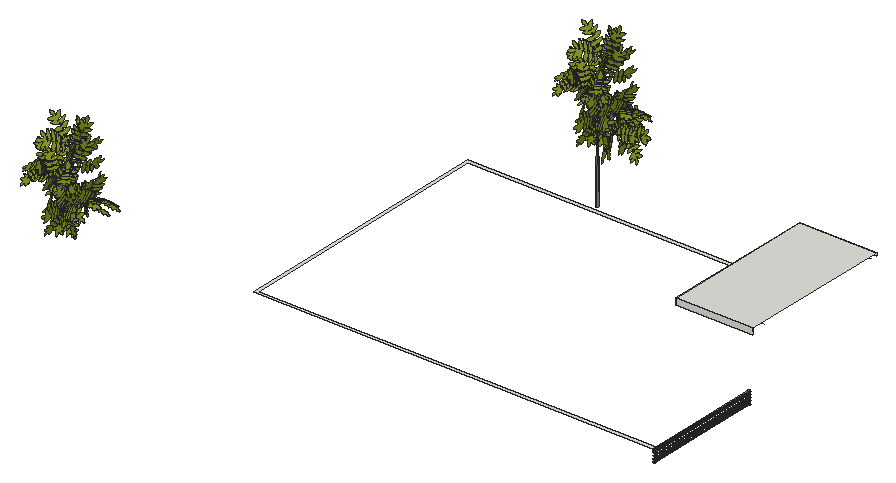
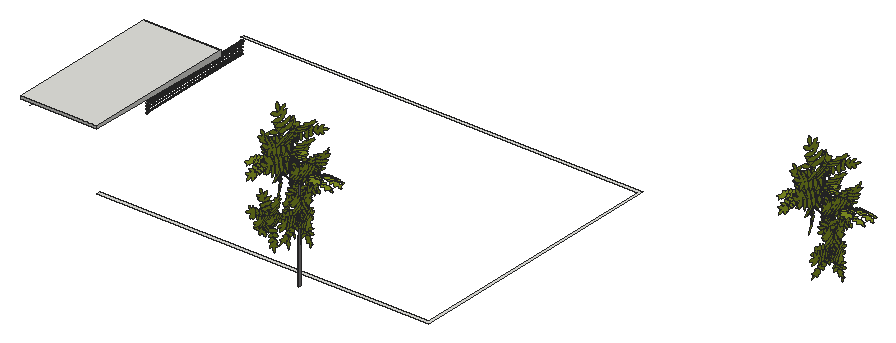
# SketchUp Ruby script. Lengths in inches.
U = 1.inch
M = Sketchup.active_model
def pt(a) = Geom::Point3d.new(a.map { |v| v * U })
def face(e, loops, mat)
  f = e.add_face(loops[0].map { |a| pt(a) })
  loops[1..].each { |l| e.add_face(l.map { |a| pt(a) }).erase! }
  f.material = f.back_material = mat if mat
  f
end
# faces: each face lists its corners as indices into pts; further lists are holes
def faces(e, pts, list, mat = nil) = list.each { |f| face(e, (f[0].is_a?(Array) ? f : [f]).map { |l| l.map { |i| pts[i] } }, mat) }
# xy, xz, yz: faces in a plane at the given z, y or x. An outline is a flat list of corners, or four numbers for a rectangle; further outlines are holes
def ring(l) = l.size == 4 ? [[l[0], l[1]], [l[2], l[1]], [l[2], l[3]], [l[0], l[3]]] : l.each_slice(2).to_a
def flat(e, list, mat, &to3) = list.each { |f| face(e, (f[0].is_a?(Array) ? f : [f]).map { |l| ring(l).map { |u, v| to3.(u, v) } }, mat) }
def xy(e, z, list, mat = nil) = flat(e, list, mat) { |x, y| [x, y, z] }
def xz(e, y, list, mat = nil) = flat(e, list, mat) { |x, z| [x, y, z] }
def yz(e, x, list, mat = nil) = flat(e, list, mat) { |y, z| [x, y, z] }
def lines(e, pts, list) = list.each { |a, b| e.add_line(pt(pts[a]), pt(pts[b])) }
# prism: a flat outline (further loops are holes) pulled along v
def prism(e, loops, v, mat = nil)
  f = face(e, loops, mat); d = Geom::Vector3d.new(v.map { |x| x * U })
  f.pushpull(f.normal.samedirection?(d) ? d.length : -d.length)
end
def box(e, o, s, mat = nil) = prism(e, [[o, [o[0] + s[0], o[1], o[2]], [o[0] + s[0], o[1] + s[1], o[2]], [o[0], o[1] + s[1], o[2]]]], [0, 0, s[2]], mat)
def at(x, y, z, deg = 0) = Geom::Transformation.translation(pt([x, y, z])) * Geom::Transformation.rotation(ORIGIN, Z_AXIS, deg.degrees)
def axes(o, x, y, z) = Geom::Transformation.new([*x, 0, *y, 0, *z, 0, *pt(o).to_a, 1])
def part(name) = M.definitions.add(name)
# library, detail: a bought-in or finely detailed component or shape, given as its bounding box
def library(name, o, s) = part(name).tap { |d| box(d.entities, o, s) }
def detail(e, o, s) = box(e.add_group.entities, o, s)
def put(e, d, t, mat = nil) = e.add_instance(d, t).tap { |i| i.material = mat if mat }
def group(e, t, mat = nil) = e.add_group.tap { |g| g.transformation = t; g.material = mat if mat }.entities
root = M.entities
M.materials.add("3D66_SU_1574822641685_001").color = [135, 150, 36]
M.materials.add("3D66_SU_1574822641883_002").color = [178, 165, 164]
M.materials.add("3D66_SU_1574822642012_003").color = [128, 125, 127]
M.materials.add("[Aluminum]").color = [150, 150, 150]
M.materials["[Aluminum]"].alpha = 0.5
c1 = part("rama-acacia")
p = [[-13.8,1.01,-1.08],[-13.61,0.91,-1.04],[-13.61,0.85,-1.06],[-14.07,0.85,-1.21],[-15.17,0.86,-1.58],[-15.95,0.92,-1.83],
  [-16.01,1,-1.83],[-16.01,1.17,-1.78],[-16.07,1.93,-1.6],[-16.4,2.73,-1.5],[-16.65,3.06,-1.5],[-17.13,4.01,-1.41],
  [-17.78,4.7,-1.44],[-18.28,5.07,-1.51],[-18.57,5.18,-1.58],[-18.91,5.47,-1.62],[-19.07,5.48,-1.67],[-19.35,5.61,-1.73],
  [-19.51,5.64,-1.78],[-19.38,5.57,-1.75],[-19.33,5.5,-1.75],[-19.31,5.23,-1.82],[-19.38,5.08,-1.89],[-19.41,4.84,-1.96],
  [-19.36,4.59,-2.01],[-19.43,4.55,-2.04],[-19.36,4.15,-2.125],[-19.21,3.7,-2.19],[-18.875,3.1,-2.24],[-18.61,2.78,-2.24],
  [-17.83,2.19,-2.13],[-17.4375,1.85,-2.09],[-17.04,1.49,-2.05],[-16.61,1.24,-1.97],[-16.17,1.0625,-1.87],[-16.06,0.95,-1.86],
  [-16.06,0.91,-1.87],[-16.32,0.9,-1.96],[-16.7,0.88,-2.1],[-17.05,0.91,-2.21],[-17.61,1.15,-2.33],[-18.06,1.29,-2.45],
  [-18.88,1.53,-2.67],[-20.25,1.46,-3.15],[-20.59,1.49,-3.26],[-20.79,1.37,-3.36],[-21.08,1.2,-3.5],[-21.28,1.22,-3.5625],
  [-21.48,0.94,-3.71],[-21.79,0.5,-3.93],[-22.02,0.17,-4.1],[-22.11,0.05,-4.16],[-22.21,-0.02,-4.21],[-22.375,-0.05,-4.28],
  [-22.375,-0.07,-4.28],[-22.18,-0.09,-4.22],[-22.11,-0.07,-4.19],[-21.78,-0.1,-4.09],[-21.6,-0.18,-4.05],[-21.52,-0.27,-4.04],
  [-21.33,-0.33,-4],[-20.94,-0.54,-3.92],[-20.6875,-0.63,-3.86],[-20.54,-0.68,-3.82],[-20.42,-0.67,-3.78],[-20.09,-0.46,-3.61],
  [-19.8,-0.24,-3.45],[-19.21,-0.02,-3.19],[-18.48,0.08,-2.92],[-17.72,0.38,-2.58],[-17.4,0.5,-2.4375],[-16.93,0.75,-2.21],
  [-16.78,0.8,-2.15],[-16.1,0.83,-1.91],[-16.0625,0.81,-1.9],[-16.08,0.77,-1.91],[-16.27,0.72,-1.99],[-16.88,0.39,-2.29],
  [-17.1875,0.15,-2.46],[-17.27,0.02,-2.52],[-17.94,-0.52,-2.89],[-17.94,-0.59,-2.91],[-18.08,-0.68,-2.99],[-18.13,-0.86,-3.05],
  [-18.56,-1.55,-3.38],[-18.71,-2.11,-3.58],[-18.79,-2.61,-3.74],[-18.86,-2.84,-3.83],[-18.87,-3.07,-3.89],[-18.84,-3.22,-3.92],
  [-18.8,-3.26,-3.92],[-18.76,-3.47,-3.96],[-18.76,-3.6,-4],[-18.67,-3.8,-4.02],[-18.61,-3.92,-4.04],[-18.58,-4.11,-4.07],
  [-18.53,-4.18,-4.08],[-18.58,-4.35,-4.14],[-18.65,-4.43,-4.18],[-18.72,-4.51,-4.23],[-18.8125,-4.51,-4.26],[-18.8125,-4.53,-4.26],
  [-18.72,-4.54,-4.24],[-18.66,-4.49,-4.21],[-18.58,-4.43,-4.16],[-18.35,-4.23,-4.03],[-18.32,-4.17,-4],[-18.22,-4.125,-3.95],
  [-18.1,-4,-3.88],[-17.79,-3.72,-3.7],[-17.68,-3.51,-3.61],[-17.32,-3.13,-3.38],[-17.24,-2.94,-3.31],[-16.78,-2.12,-2.93],
  [-16.48,-1.78,-2.73],[-16.3,-1.28,-2.54],[-16.05,-0.75,-2.3125],[-15.89,-0.2,-2.11],[-15.89,0.39,-1.95],[-15.96,0.79,-1.87],
  [-15.91,0.82,-1.84],[-15.27,0.8,-1.63],[-14.18,0.76,-1.27],[-13.78,0.73,-1.15],[-13.78,0.67,-1.16],[-14.23,0.54,-1.35],
  [-14.65,0.33,-1.55],[-14.97,0.02,-1.74],[-15.25,-0.36,-1.9375],[-15.57,-0.72,-2.14],[-15.96,-1.64,-2.52],[-16.2,-2.51,-2.84],
  [-16.2,-3.12,-3],[-16.14,-3.41,-3.06],[-16.1,-3.75,-3.14],[-16.1,-4.09,-3.23],[-16.2,-4.25,-3.3],[-16.2,-4.28,-3.3125],
  [-16.08,-4.19,-3.24],[-15.98,-4.08,-3.18],[-15.96,-3.94,-3.14],[-15.96,-3.8125,-3.1],[-15.9,-3.72,-3.06],[-15.68,-3.55,-2.9375],
  [-15.51,-3.49,-2.86],[-15.3,-3.33,-2.75],[-15.23,-3.17,-2.68],[-15.01,-3.03,-2.57],[-14.875,-2.83,-2.47],[-14.6,-2.59,-2.3125],
  [-14.4,-2.27,-2.16],[-14.12,-1.6,-1.89],[-13.91,-1.1,-1.68],[-13.67,-0.83,-1.53],[-13.53,-0.45,-1.38],[-13.53,0.67,-1.08],
  [-13.53,0.69,-1.07],[-13.38,0.86,-0.98],[-13.38,0.92,-0.96],[-13.32,1.03,-0.91],[-13.32,1.35,-0.82],[-13.28,1.49,-0.77],
  [-13.28,1.99,-0.64],[-13.44,2.67,-0.51],[-13.72,3.31,-0.43],[-13.93,3.71,-0.4],[-14.1,4.39,-0.27],[-14.5625,5.06,-0.25],
  [-14.89,5.62,-0.21],[-15.33,6.1,-0.23],[-15.65,6.8,-0.15],[-15.79,6.89,-0.18],[-15.61,6.52,-0.22],[-15.51,6.32,-0.24],
  [-15.45,6.28,-0.23],[-15.52,6,-0.32],[-15.63,5.6875,-0.45],[-15.77,4.97,-0.68],[-15.7,4.25,-0.85],[-15.46,3,-1.11],
  [-15,2.03,-1.21],[-14.3,1.29,-1.17],[-12.41,6.01,0.65],[-12.44,6.14,0.68],[-12.41,6.29,0.73],[-12.43,6.29,0.73],
  [-12.44,6.26,0.72],[-12.47,6.15,0.68],[-12.49,6.07,0.66],[-12.57,5.75,0.55],[-12.67,5.36,0.43],[-12.79,4.875,0.28],
  [-12.83,4.52,0.18],[-12.83,3.99,0.04],[-12.73,3.11,-0.18],[-12.58,2.52,-0.3125],[-12.3,1.97,-0.41],[-11.88,1.51,-0.46],
  [-11.37,1.0625,-0.48],[-10.75,0.75,-0.45],[-10.75,0.68,-0.47],[-12.55,0.7,-0.79],[-13.21,0.79,-0.89],[-13.2,0.67,-0.92],
  [-12.56,0.62,-0.82],[-11.15,0.56,-0.58],[-10.79,0.54,-0.52],[-10.72,0.52,-0.51],[-10.72,0.5,-0.52],[-10.87,0.47,-0.55],
  [-11.14,0.41,-0.62],[-11.39,0.27,-0.7],[-11.625,-0.01,-0.82],[-11.8,-0.43,-0.96],[-11.83,-0.57,-1],[-12.02,-1.08,-1.17],
  [-12.1,-1.39,-1.27],[-12.17,-1.95,-1.4375],[-12.17,-2.77,-1.65],[-12.09,-3.59,-1.86],[-11.86,-4.26,-2],[-11.8125,-4.4,-2.03],
  [-11.84,-4.49,-2.05],[-11.91,-4.6,-2.1],[-11.97,-4.65,-2.12],[-11.98,-4.67,-2.13],[-11.92,-4.65,-2.11],[-11.84,-4.59,-2.08],
  [-11.77,-4.52,-2.05],[-11.74,-4.47,-2.03],[-11.37,-4.3125,-1.92],[-10.95,-4.0625,-1.78],[-10.82,-3.89,-1.71],[-10.64,-3.57,-1.59],
  [-10.41,-3.05,-1.41],[-10.27,-2.73,-1.3],[-10.07,-1.88,-1.03],[-10.15,-0.71,-0.73],[-10.31,-0.1,-0.6],[-10.5,0.4,-0.5],
  [-10.5,0.48,-0.48],[-10.44,0.53,-0.45],[-10.39,0.64,-0.42],[-10.52,0.73,-0.42],[-10.44,0.93,-0.35],[-10.44,1.2,-0.28],
  [-10.32,1.47,-0.18],[-10.48,2.6875,0.12],[-10.43,2.96,0.2],[-10.75,3.87,0.38],[-11.26,4.93,0.57],[-11.8,5.54,0.64],
  [-12.37,5.93,0.64],[-7.78,0.19,-0.06],[-7.78,0.25,-0.04],[-7.75,0.39,0],[-7.89,0.4,-0.02],[-7.96,0.46,-0.02],
  [-7.96,0.49,-0.01],[-7.76,0.62,0.06],[-7.53,0.99,0.2],[-7.31,1.78,0.45],[-7.31,2.74,0.71],[-7.63,3.6875,0.9],
  [-8.02,4.57,1.07],[-8.66,5.23,1.13],[-8.83,5.4,1.14],[-8.92,5.54,1.16],[-9.1,5.64,1.16],[-9.08,5.6,1.15],
  [-9.02,5.56,1.15],[-8.94,5.46,1.14],[-8.9,5.37,1.12],[-8.9375,5.25,1.08],[-9.14,4.92,0.96],[-9.31,4.5625,0.83],
  [-9.39,3.73,0.6],[-9.44,2.76,0.32],[-9.23,1.59,0.05],[-8.82,0.9,-0.06],[-8.36,0.59,-0.0625],[-8.14,0.51,-0.04],
  [-8.05,0.48,-0.03],[-8.05,0.46,-0.04],[-8.12,0.43,-0.06],[-10.1,0.49,-0.4],[-8.22,0.3125,-0.11],[-8.22,0.25,-0.125],
  [-8.53,0.13,-0.21],[-8.8,-0.16,-0.34],[-8.96,-0.61,-0.49],[-8.96,-0.87,-0.56],[-9.16,-1.42,-0.74],[-9.13,-1.77,-0.83],
  [-9.09,-1.83,-0.84],[-9.125,-1.92,-0.87],[-9.125,-2.13,-0.93],[-9.08,-2.23,-0.95],[-9.15,-2.39,-1],[-9.11,-2.67,-1.07],
  [-9.03,-2.86,-1.11],[-9.07,-3.03,-1.16],[-8.97,-3.23,-1.19],[-8.93,-3.44,-1.24],[-8.93,-3.71,-1.32],[-8.79,-4.05,-1.38],
  [-8.7,-4.25,-1.42],[-8.7,-4.39,-1.46],[-8.76,-4.53,-1.5],[-8.77,-4.65,-1.54],[-8.64,-4.55,-1.49],[-8.27,-4.22,-1.33],
  [-8.1875,-4.06,-1.27],[-8.07,-3.98,-1.23],[-7.98,-3.79,-1.17],[-7.79,-3.59,-1.08],[-7.64,-3.3,-0.97],[-7.64,-3.25,-0.96],
  [-7.59,-3.21,-0.9375],[-7.52,-2.93,-0.85],[-7.52,-2.85,-0.83],[-7.47,-2.81,-0.81],[-7.3,-2.09,-0.59],[-7.32,-2.01,-0.57],
  [-7.27,-1.95,-0.54],[-7.1875,-1.57,-0.42],[-7.17,-1.46,-0.39],[-7.17,-1.16,-0.3125],[-7.23,-0.61,-0.17],[-7.49,-0.15,-0.1],
  [-13.39,-0.07,-1.23],[-13.39,0.25,-1.14],[-13.49,0.5625,-1.09],[-4.5625,0.33,0.09],[-4.22,0.49,0.13],[-4,0.7,0.1875],
  [-3.86,0.99,0.26],[-3.77,1.41,0.38],[-3.7,1.73,0.46],[-3.77,1.99,0.53],[-3.85,2.17,0.58],[-3.88,2.57,0.6875],
  [-3.98,2.9,0.78],[-4.0625,2.97,0.8],[-4.1,3.14,0.84],[-4.1875,3.25,0.87],[-4.27,3.55,0.95],[-4.31,3.71,0.99],
  [-4.42,3.9,1.04],[-4.625,4.2,1.125],[-4.72,4.39,1.18],[-4.89,4.57,1.23],[-4.98,4.73,1.27],[-5,4.72,1.26],
  [-5.01,4.51,1.21],[-4.96,4.32,1.16],[-4.97,4.27,1.14],[-5.14,3.78,1.01],[-5.3,3.39,0.91],[-5.44,2.76,0.74],
  [-5.5,2.09,0.56],[-5.57,1.78,0.48],[-5.57,1.42,0.38],[-5.57,1.09,0.29],[-5.47,0.72,0.19],[-5.22,0.44,0.12],
  [-4.93,0.27,0.07],[-4.76,0.22,0.06],[-4.76,0.18,0.05],[-4.83,0.16,0.04],[-5.26,0,0],[-5.34,-0.04,-0.01],
  [-5.47,-0.22,-0.06],[-5.51,-0.6,-0.16],[-5.42,-1.09,-0.29],[-5.28,-1.49,-0.4],[-5.21,-1.87,-0.5],[-5.11,-2.15,-0.57],
  [-5.08,-2.34,-0.63],[-5.01,-2.47,-0.66],[-4.96,-2.69,-0.72],[-4.86,-2.9375,-0.79],[-4.84,-3.07,-0.82],[-4.77,-3.18,-0.85],
  [-4.74,-3.43,-0.92],[-4.7,-3.71,-0.99],[-4.62,-3.89,-1.04],[-4.58,-3.98,-1.07],[-4.58,-3.83,-1.03],[-4.51,-3.67,-0.98],
  [-4.3,-3.32,-0.89],[-4.16,-3.09,-0.83],[-4.16,-2.98,-0.8],[-4.11,-2.92,-0.78],[-4.02,-2.8,-0.75],[-3.95,-2.59,-0.69],
  [-3.95,-2.33,-0.625],[-3.86,-2.26,-0.6],[-3.86,-2.02,-0.54],[-3.86,-1.44,-0.39],[-3.94,-1.22,-0.33],[-3.94,-1.08,-0.29],
  [-4,-0.96,-0.26],[-4,-0.87,-0.23],[-4.0625,-0.8125,-0.22],[-4.16,-0.54,-0.14],[-4.39,-0.24,-0.06],[-4.61,-0.08,-0.02],
  [-4.77,-0.03,-0.01],[-4.77,-0.01,0],[-4.65,-0.01,0],[-4.61,0.19,0.05],[-4.66,0.23,0.0625],[-4.63,0.29,0.08],
  [-4.07,0.17,0.04],[0,-0.24,-0.06],[0,0,0],[-0.5,0.04,0.01],[-1.58,0.08,0.02]]
faces(c1.entities,p,[[0,1,2,3,4,5,6,7,8,9,10,11,12,13,14,15,16,17,18,19,20,21,22,23,24,25,26,27,28,29,30,31,32,33,34,35,36,37,38,39,40,41,42,43,44,45,46,47,48,49,50,51,52,53,54,55,56,57,58,59,60,61,62,63,64,65,66,67,68,69,70,71,72,73,74,75,76,77,78,79,80,81,82,83,84,85,86,87,88,89,90,91,92,93,94,95,96,97,98,99,100,101,102,103,104,105,106,107,108,109,110,111,112,113,114,115,116,117,118,119,120,121,122,123,124,125,126,127,128,129,130,131,132,133,134,135,136,137,138,139,140,141,142,143,144,145,146,147,148,149,150,151,152,153,154,155,156,157,158,159,160,161,162,163,164,165,166,167,168,169,170,171,172,173,174,175,176,177,178,179,180,181],[182,183,184,185,186,187,188,189,190,191,192,193,194,195,196,197,198,199,200,201,202,203,204,205,206,207,208,209,210,211,212,213,214,215,216,217,218,219,220,221,222,223,224,225,226,227,228,229,230,231,232,233,234,235,236,237,238,239,240,241,242,243,244,245,246,247,248,249,250,251,252],[253,254,255,256,257,258,259,260,261,262,263,264,265,266,267,268,269,270,271,272,273,274,275,276,277,278,279,280,281,282,283,284,242,241,285,286,287,288,289,290,291,292,293,294,295,296,297,298,299,300,301,302,303,304,305,306,307,308,309,310,311,312,313,314,315,316,317,318,319,320,321,322,323,324,325,326,327,328,329],[154,330,331,332,155],[333,334,335,336,337,338,339,340,341,342,343,344,345,346,347,348,349,350,351,352,353,354,355,356,357,358,359,360,361,362,363,364,365,366,367,368,369,370,371,372,373,374,375,376,377,378,379,380,381,382,383,384,385,386,387,388,389,390,391,392,393,394,395,396,397,398,399,400,401,402,403,404,405,406,407,408,409,410,411,412,413],[156,203,157],[202,157,203],[414,411,410,415,416,417,418],
  [254,370,255],[369,255,370]],"3D66_SU_1574822641685_001")
c2 = part("ramas")
put(c2.entities,c1,axes([0.11,0.06,-0.22],[-0.42655,-0.79206,-0.43668],[0.22445,0.37501,-0.89944],[0.87617,-0.48167,0.01782]))
put(c2.entities,c1,axes([0.14,0.21,0.02],[0.24321,-0.08852,-0.96593],[0.34202,0.93969,0],[0.90767,-0.33037,0.25882]))
put(c2.entities,c1,at(0,0.24,0.06))
put(c2.entities,c1,axes([0.11,0.45,0.57],[-0.42655,0.68302,0.5929],[0.22445,-0.55509,0.80093],[0.87617,0.47472,0.08347]))
put(c2.entities,c1,axes([0.11,0.73,0.01],[-0.42655,0.88928,-0.16503],[0.22445,0.28083,0.93314],[0.87617,0.36099,-0.31939]))
c3 = part("rama principal")
put(c3.entities,c1,axes([-20.25,-0.15,12.84],[0.38818,-0.89018,-0.23852],[0.89018,0.42916,-0.15296],[0.23852,-0.15296,0.95902]))
put(c3.entities,c1,at(-20.48,0,12.88))
put(c3.entities,c1,axes([-20.6875,-0.1,12.85],[0.57358,0.79124,0.21201],[-0.79124,0.60214,-0.10661],[-0.21201,-0.10661,0.97144]))
put(c3.entities,c1,axes([-20.375,-0.01,13.02],[-0.37792,0.77975,-0.49916],[-0.65887,0.15226,0.73669],[0.65043,0.60729,0.45621]))
put(c3.entities,c1,axes([-20.34,-0.04,12.83],[0.24321,-0.08852,-0.96593],[0.34202,0.93969,0],[0.90767,-0.33037,0.25882]))
put(c3.entities,c1,axes([-20.375,-0.18,12.6],[-0.42655,-0.79206,-0.43668],[0.22445,0.37501,-0.89944],[0.87617,-0.48167,0.01782]))
put(c3.entities,c2,at(-11.43,0,7.77))
g1 = group(c3.entities,at(0,0.2,0),"3D66_SU_1574822641883_002")
xz(g1,0.1,[[-0.15,-0.08,-3.26,5.59,-11.5,7.61,-18.23,12.71,-20.48,12.71,-20.48,13.05,-18.11,13.05,-11.35,7.92,-3.03,5.89,0.15,0.08]])
yz(g1,-20.48,[[0.1,12.71,-0.2,12.88,0.1,13.05]])
p = [[-0.15,0.1,-0.08],[0,-0.2,0],[-3.15,-0.2,5.74],[-3.26,0.1,5.59],[0.15,0.1,0.08],[-3.03,0.1,5.89],
  [-11.43,-0.2,7.77],[-11.5,0.1,7.61],[-11.35,0.1,7.92],[-18.17,-0.2,12.88],[-18.23,0.1,12.71],[-18.11,0.1,13.05],
  [-20.48,-0.2,12.88],[-20.48,0.1,12.71],[-20.48,0.1,13.05]]
faces(g1,p,[[0,1,2,3],[0,4,1],[1,4,5,2],[3,2,6,7],[2,5,8,6],[7,6,9,10],[6,8,11,9],[10,9,12,13],
  [9,11,14,12]])
xy(root,137.55,[[869.01,117.53,869.09,278.08]],"[Aluminum]")
xy(root,139.54,[[869.09,117.53,869.17,278.08]],"[Aluminum]")
xy(root,141.49,[[869.01,117.53,869.09,278.08]],"[Aluminum]")
xy(root,143.48,[[869.09,117.53,869.17,278.08]],"[Aluminum]")
xy(root,145.43,[[869.01,117.53,869.09,278.08]],"[Aluminum]")
xy(root,147.42,[[869.09,117.53,869.17,278.08]],"[Aluminum]")
xy(root,149.37,[[869.01,117.53,869.09,278.08]],"[Aluminum]")
xy(root,151.36,[[869.09,117.53,869.17,278.08]],"[Aluminum]")
xy(root,158.24,[[334.375,113.59,871.06,113.59,871.06,117.53,338.3125,117.53,338.3125,468.87,779.5,468.87,779.5,473.59,334.375,473.59]])
xy(root,239.94,[[779.5,266.28,882.86,473.59]])
xz(root,266.28,[[779.5,231.94,882.8,239.94]])
xz(root,278.08,[[869.01,137.55,868.75,137.6,868.52,137.72,868.33,137.9,868.19,138.12,868.11,138.37,868.09,138.63,868.15,138.88,868.27,139.11,868.44,139.31,868.66,139.45,868.91,139.53,869.09,139.54,869.17,139.54,869.43,139.49,869.66,139.37,869.85,139.19,869.99,138.97,870.07,138.72,870.09,138.46,870.03,138.21,869.91,137.98,869.74,137.78,869.52,137.64,869.27,137.5625,869.09,137.55],[869.01,141.49,868.75,141.54,868.52,141.66,868.33,141.84,868.19,142.06,868.11,142.31,868.09,142.57,868.15,142.82,868.27,143.05,868.44,143.25,868.66,143.39,868.91,143.47,869.09,143.48,869.17,143.48,869.43,143.43,869.66,143.31,869.85,143.13,869.99,142.91,870.07,142.66,870.09,142.4,870.03,142.15,869.91,141.92,869.74,141.72,869.52,141.58,869.27,141.5,869.09,141.49],[869.01,145.43,868.75,145.49,868.52,145.61,868.33,145.78,868.19,146,868.11,146.25,868.09,146.51,868.15,146.77,868.27,147,868.44,147.19,868.66,147.33,868.91,147.41,869.09,147.42,869.17,147.42,869.43,147.37,869.66,147.25,869.85,147.07,869.99,146.85,870.07,146.61,870.09,146.34,870.03,146.09,869.91,145.86,869.74,145.66,869.52,145.52,869.27,145.44,869.09,145.43],[869.01,149.37,868.75,149.42,868.52,149.54,868.33,149.72,868.19,149.9375,868.11,150.1875,868.09,150.45,868.15,150.7,868.27,150.93,868.44,151.13,868.66,151.27,868.91,151.35,869.09,151.36,869.17,151.36,869.43,151.31,869.66,151.1875,869.85,151.01,869.99,150.79,870.07,150.54,870.09,150.28,870.03,150.03,869.91,149.8,869.74,149.6,869.52,149.46,869.27,149.38,869.09,149.37],[869.09,153.3,868.83,153.34,868.59,153.4375,868.38,153.6,868.22,153.8,868.125,154.05,868.09,154.3,868.125,154.5625,868.22,154.8,868.38,155.01,868.59,155.17,868.83,155.27,869.09,155.3,869.35,155.27,869.59,155.17,869.8,155.01,869.96,154.8,870.06,154.5625,870.09,154.3,870.06,154.05,869.96,153.8,869.8,153.6,869.59,153.4375,869.35,153.34]])
xz(root,473.59,[[779.5,236,882.86,239.94]])
yz(root,779.5,[[266.28,231.94,266.28,239.94,473.59,239.94,473.59,236]])
yz(root,871.06,[[286.08,231.94,465.59,236]])
p = [[869.01,117.53,137.55],[868.75,117.53,137.6],[868.75,278.08,137.6],[869.01,278.08,137.55],[868.52,117.53,137.72],[868.52,278.08,137.72],
  [869.27,117.53,137.5625],[869.09,117.53,137.55],[869.09,278.08,137.55],[869.27,278.08,137.5625],[869.52,117.53,137.64],[869.52,278.08,137.64],
  [869.74,117.53,137.78],[869.74,278.08,137.78],[868.33,117.53,137.9],[868.33,278.08,137.9],[869.91,117.53,137.98],[869.91,278.08,137.98],
  [868.19,117.53,138.12],[868.19,278.08,138.12],[870.03,117.53,138.21],[870.03,278.08,138.21],[868.11,117.53,138.37],[868.11,278.08,138.37],
  [870.09,117.53,138.46],[870.09,278.08,138.46],[868.09,117.53,138.63],[868.09,278.08,138.63],[870.07,117.53,138.72],[870.07,278.08,138.72],
  [868.15,117.53,138.88],[868.15,278.08,138.88],[869.99,117.53,138.97],[869.99,278.08,138.97],[868.27,117.53,139.11],[868.27,278.08,139.11],
  [869.85,117.53,139.19],[869.85,278.08,139.19],[868.44,117.53,139.31],[868.44,278.08,139.31],[869.66,117.53,139.37],[869.66,278.08,139.37],
  [868.66,117.53,139.45],[868.66,278.08,139.45],[868.91,117.53,139.53],[868.91,278.08,139.53],[869.43,117.53,139.49],[869.43,278.08,139.49],
  [869.09,117.53,139.54],[869.09,278.08,139.54],[869.17,117.53,139.54],[869.17,278.08,139.54],[868.75,117.53,141.54],[868.52,117.53,141.66],
  [868.52,278.08,141.66],[868.75,278.08,141.54],[869.01,117.53,141.49],[869.01,278.08,141.49],[869.27,117.53,141.5],[869.09,117.53,141.49],
  [869.09,278.08,141.49],[869.27,278.08,141.5],[869.52,117.53,141.58],[869.52,278.08,141.58],[869.74,117.53,141.72],[869.74,278.08,141.72],
  [868.33,117.53,141.84],[868.33,278.08,141.84],[869.91,117.53,141.92],[869.91,278.08,141.92],[868.19,117.53,142.06],[868.19,278.08,142.06],
  [870.03,117.53,142.15],[870.03,278.08,142.15],[868.11,117.53,142.31],[868.11,278.08,142.31],[870.09,117.53,142.4],[870.09,278.08,142.4],
  [868.09,117.53,142.57],[868.09,278.08,142.57],[870.07,117.53,142.66],[870.07,278.08,142.66],[868.15,117.53,142.82],[868.15,278.08,142.82],
  [869.99,117.53,142.91],[869.99,278.08,142.91],[868.27,117.53,143.05],[868.27,278.08,143.05],[869.85,117.53,143.13],[869.85,278.08,143.13],
  [868.44,117.53,143.25],[868.44,278.08,143.25],[869.66,117.53,143.31],[869.66,278.08,143.31],[868.66,117.53,143.39],[868.66,278.08,143.39],
  [869.43,117.53,143.43],[869.43,278.08,143.43],[868.91,117.53,143.47],[868.91,278.08,143.47],[869.17,117.53,143.48],[869.17,278.08,143.48],
  [869.09,117.53,143.48],[869.09,278.08,143.48],[869.01,117.53,145.43],[868.75,117.53,145.49],[868.75,278.08,145.49],[869.01,278.08,145.43],
  [869.27,117.53,145.44],[869.09,117.53,145.43],[869.09,278.08,145.43],[869.27,278.08,145.44],[869.52,117.53,145.52],[869.52,278.08,145.52],
  [868.52,117.53,145.61],[868.52,278.08,145.61],[869.74,117.53,145.66],[869.74,278.08,145.66],[868.33,117.53,145.78],[868.33,278.08,145.78],
  [869.91,117.53,145.86],[869.91,278.08,145.86],[868.19,117.53,146],[868.19,278.08,146],[870.03,117.53,146.09],[870.03,278.08,146.09],
  [868.11,117.53,146.25],[868.11,278.08,146.25],[870.09,117.53,146.34],[870.09,278.08,146.34],[868.09,117.53,146.51],[868.09,278.08,146.51],
  [870.07,117.53,146.61],[870.07,278.08,146.61],[868.15,117.53,146.77],[868.15,278.08,146.77],[869.99,117.53,146.85],[869.99,278.08,146.85],
  [868.27,117.53,147],[868.27,278.08,147],[869.85,117.53,147.07],[869.85,278.08,147.07],[868.44,117.53,147.19],[868.44,278.08,147.19],
  [869.66,117.53,147.25],[869.66,278.08,147.25],[868.66,117.53,147.33],[868.66,278.08,147.33],[869.43,117.53,147.37],[869.43,278.08,147.37],
  [868.91,117.53,147.41],[868.91,278.08,147.41],[869.09,117.53,147.42],[869.09,278.08,147.42],[869.17,117.53,147.42],[869.17,278.08,147.42],
  [868.75,117.53,149.42],[868.52,117.53,149.54],[868.52,278.08,149.54],[868.75,278.08,149.42],[869.01,117.53,149.37],[869.01,278.08,149.37],
  [869.27,117.53,149.38],[869.09,117.53,149.37],[869.09,278.08,149.37],[869.27,278.08,149.38],[869.52,117.53,149.46],[869.52,278.08,149.46],
  [868.33,117.53,149.72],[868.33,278.08,149.72],[869.74,117.53,149.6],[869.74,278.08,149.6],[869.91,117.53,149.8],[869.91,278.08,149.8],
  [868.19,117.53,149.9375],[868.19,278.08,149.9375],[870.03,117.53,150.03],[870.03,278.08,150.03],[868.11,117.53,150.1875],[868.11,278.08,150.1875],
  [870.09,117.53,150.28],[870.09,278.08,150.28],[868.09,117.53,150.45],[868.09,278.08,150.45],[870.07,117.53,150.54],[870.07,278.08,150.54],
  [868.15,117.53,150.7],[868.15,278.08,150.7],[869.99,117.53,150.79],[869.99,278.08,150.79],[868.27,117.53,150.93],[868.27,278.08,150.93],
  [869.85,117.53,151.01],[869.85,278.08,151.01],[868.44,117.53,151.13],[868.44,278.08,151.13],[869.66,117.53,151.1875],[869.66,278.08,151.1875],
  [868.66,117.53,151.27],[868.66,278.08,151.27],[869.43,117.53,151.31],[869.43,278.08,151.31],[868.91,117.53,151.35],[868.91,278.08,151.35],
  [869.09,117.53,151.36],[869.09,278.08,151.36],[869.17,117.53,151.36],[869.17,278.08,151.36],[868.83,117.53,153.34],[868.59,117.53,153.4375],
  [868.59,278.08,153.4375],[868.83,278.08,153.34],[869.09,117.53,153.3],[869.09,278.08,153.3],[869.35,117.53,153.34],[869.35,278.08,153.34],
  [869.59,117.53,153.4375],[869.59,278.08,153.4375],[868.38,117.53,153.6],[868.38,278.08,153.6],[869.8,117.53,153.6],[869.8,278.08,153.6],
  [868.22,117.53,153.8],[868.22,278.08,153.8],[869.96,117.53,153.8],[869.96,278.08,153.8],[868.125,117.53,154.05],[868.125,278.08,154.05],
  [870.06,117.53,154.05],[870.06,278.08,154.05],[868.09,117.53,154.3],[868.09,278.08,154.3],[870.09,117.53,154.3],[870.09,278.08,154.3],
  [868.125,117.53,154.5625],[868.125,278.08,154.5625],[870.06,117.53,154.5625],[870.06,278.08,154.5625],[868.22,117.53,154.8],[868.22,278.08,154.8],
  [869.96,117.53,154.8],[869.96,278.08,154.8],[868.38,117.53,155.01],[868.38,278.08,155.01],[869.8,117.53,155.01],[869.8,278.08,155.01],
  [868.59,117.53,155.17],[868.59,278.08,155.17],[869.59,117.53,155.17],[869.59,278.08,155.17],[868.83,117.53,155.27],[868.83,278.08,155.27],
  [869.35,117.53,155.27],[869.35,278.08,155.27],[869.09,117.53,155.3],[869.09,278.08,155.3],[871.06,278.08,231.94],[871.06,286.08,231.94],
  [871.06,465.59,231.94],[871.06,473.59,231.94],[871.06,465.59,236],[882.86,465.59,236],[871.06,286.08,236],[882.86,286.08,236],
  [882.86,266.28,239.94],[882.86,266.28,236]]
faces(root,p,[[0,1,2,3],[1,4,5,2],[6,7,8,9],[10,6,9,11],[12,10,11,13],[4,14,15,5],[16,12,13,17],[14,18,19,15],
  [20,16,17,21],[18,22,23,19],[24,20,21,25],[22,26,27,23],[28,24,25,29],[26,30,31,27],[32,28,29,33],[30,34,35,31],
  [36,32,33,37],[34,38,39,35],[40,36,37,41],[38,42,43,39],[42,44,45,43],[46,40,41,47],[44,48,49,45],[50,46,47,51],
  [52,53,54,55],[56,52,55,57],[58,59,60,61],[62,58,61,63],[64,62,63,65],[53,66,67,54],[68,64,65,69],[66,70,71,67],
  [72,68,69,73],[70,74,75,71],[76,72,73,77],[74,78,79,75],[80,76,77,81],[78,82,83,79],[84,80,81,85],[82,86,87,83],
  [88,84,85,89],[86,90,91,87],[92,88,89,93],[90,94,95,91],[96,92,93,97],[94,98,99,95],[100,96,97,101],[98,102,103,99],
  [104,105,106,107],[108,109,110,111],[112,108,111,113],[105,114,115,106],[116,112,113,117],[114,118,119,115],[120,116,117,121],[118,122,123,119],
  [124,120,121,125],[122,126,127,123],[128,124,125,129],[126,130,131,127],[132,128,129,133],[130,134,135,131],[136,132,133,137],[134,138,139,135],
  [140,136,137,141],[138,142,143,139],[144,140,141,145],[142,146,147,143],[148,144,145,149],[146,150,151,147],[150,152,153,151],[154,148,149,155],
  [156,157,158,159],[160,156,159,161],[162,163,164,165],[166,162,165,167],[157,168,169,158],[170,166,167,171],[172,170,171,173],[168,174,175,169],
  [176,172,173,177],[174,178,179,175],[180,176,177,181],[178,182,183,179],[184,180,181,185],[182,186,187,183],[188,184,185,189],[186,190,191,187],
  [192,188,189,193],[190,194,195,191],[196,192,193,197],[194,198,199,195],[200,196,197,201],[198,202,203,199],[202,204,205,203],[206,200,201,207],
  [214,212,213,215],[216,214,215,217],[220,216,217,221],[224,220,221,225],[228,224,225,229],[232,228,229,233],[236,232,233,237],[240,236,237,241],
  [244,240,241,245],[248,244,245,249],[252,248,249,253],[254,252,253,255]],"[Aluminum]")
faces(root,p,[[208,209,210,211],[212,208,211,213],[209,218,219,210],[218,222,223,219],[222,226,227,223],[226,230,231,227],[230,234,235,231],[234,238,239,235],
  [238,242,243,239],[242,246,247,243],[246,250,251,247],[250,254,255,251]])
lines(root,p,[[256,257],[258,259],[260,261],[262,263],[264,265]])
put(root,c3,axes([98.03,93.39,176.34],[0.02343,-1.2198,0],[0,0,1.6799],[-1.30979,-0.02182,0]))
g2 = group(root,at(496.7,488.17,50.32))
xy(g2,102.61,[[-0.92,-1.17,-0.92,1.17,1.3125,0]],"3D66_SU_1574822642012_003")
xy(g2,224.33,[[-0.4,-0.625,0.79,0,-0.4,0.625]],"3D66_SU_1574822642012_003")
p = [[-0.4,-0.625,224.33],[-0.4,0.625,224.33],[-0.92,1.17,102.61],[-0.92,-1.17,102.61],[1.3125,0,102.61],[0.79,0,224.33]]
faces(g2,p,[[0,1,2,3],[4,5,0,3],[2,1,5,4]],"3D66_SU_1574822642012_003")
put(root,c3,axes([97.7,92.51,199.73],[0.0056,1.21999,0],[0,0,1.6799],[1.30999,-0.00522,0]))
put(root,c3,axes([113.72,86.34,189.71],[-1.28631,-0.23095,0],[0.24798,-1.19794,0],[0,0,1.6799]))
put(root,c3,axes([98.59,91.79,200.23],[1.31,0,0],[0,1.22,0],[0,0,1.6799]))
put(root,c3,axes([101.31,99.85,203.19],[0.97142,0,-1.79374],[0,1.586,0],[1.39877,0,1.24571]))
put(root,c3,axes([496.94,487.94,237.88],[-1.22279,-0.43771,0],[0,0,1.6799],[-0.47,1.13878,0]))
put(root,c3,axes([496.3,488.61,250.76],[0.02343,-1.2198,0],[0,0,1.6799],[-1.30979,-0.02182,0]))
put(root,c3,axes([495.98,487.73,274.15],[0.0056,1.21999,0],[0,0,1.6799],[1.30999,-0.00522,0]))
put(root,c3,axes([511.99,481.55,264.13],[-1.28631,-0.23095,0],[0.24798,-1.19794,0],[0,0,1.6799]))
put(root,c3,axes([496.87,487,274.65],[1.31,0,0],[0,1.22,0],[0,0,1.6799]))
put(root,c3,axes([499.58,495.07,277.61],[0.97142,0,-1.79374],[0,1.586,0],[1.39877,0,1.24571]))
